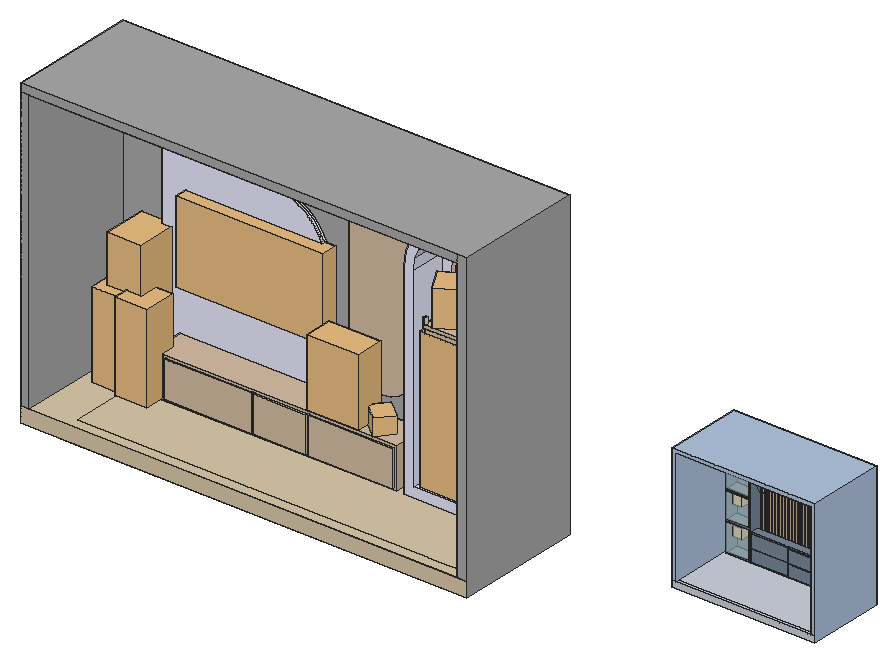
# SketchUp Ruby script. Lengths in inches.
U = 1.inch
M = Sketchup.active_model
def pt(a) = Geom::Point3d.new(a.map { |v| v * U })
def face(e, loops, mat)
  f = e.add_face(loops[0].map { |a| pt(a) })
  loops[1..].each { |l| e.add_face(l.map { |a| pt(a) }).erase! }
  f.material = f.back_material = mat if mat
  f
end
# faces: each face lists its corners as indices into pts; further lists are holes
def faces(e, pts, list, mat = nil) = list.each { |f| face(e, (f[0].is_a?(Array) ? f : [f]).map { |l| l.map { |i| pts[i] } }, mat) }
# xy, xz, yz: faces in a plane at the given z, y or x. An outline is a flat list of corners, or four numbers for a rectangle; further outlines are holes
def ring(l) = l.size == 4 ? [[l[0], l[1]], [l[2], l[1]], [l[2], l[3]], [l[0], l[3]]] : l.each_slice(2).to_a
def flat(e, list, mat, &to3) = list.each { |f| face(e, (f[0].is_a?(Array) ? f : [f]).map { |l| ring(l).map { |u, v| to3.(u, v) } }, mat) }
def xy(e, z, list, mat = nil) = flat(e, list, mat) { |x, y| [x, y, z] }
def xz(e, y, list, mat = nil) = flat(e, list, mat) { |x, z| [x, y, z] }
def yz(e, x, list, mat = nil) = flat(e, list, mat) { |y, z| [x, y, z] }
def lines(e, pts, list) = list.each { |a, b| e.add_line(pt(pts[a]), pt(pts[b])) }
# prism: a flat outline (further loops are holes) pulled along v
def prism(e, loops, v, mat = nil)
  f = face(e, loops, mat); d = Geom::Vector3d.new(v.map { |x| x * U })
  f.pushpull(f.normal.samedirection?(d) ? d.length : -d.length)
end
def box(e, o, s, mat = nil) = prism(e, [[o, [o[0] + s[0], o[1], o[2]], [o[0] + s[0], o[1] + s[1], o[2]], [o[0], o[1] + s[1], o[2]]]], [0, 0, s[2]], mat)
def at(x, y, z, deg = 0) = Geom::Transformation.translation(pt([x, y, z])) * Geom::Transformation.rotation(ORIGIN, Z_AXIS, deg.degrees)
def axes(o, x, y, z) = Geom::Transformation.new([*x, 0, *y, 0, *z, 0, *pt(o).to_a, 1])
def part(name) = M.definitions.add(name)
# library, detail: a bought-in or finely detailed component or shape, given as its bounding box
def library(name, o, s) = part(name).tap { |d| box(d.entities, o, s) }
def detail(e, o, s) = box(e.add_group.entities, o, s)
def put(e, d, t, mat = nil) = e.add_instance(d, t).tap { |i| i.material = mat if mat }
def group(e, t, mat = nil) = e.add_group.tap { |g| g.transformation = t; g.material = mat if mat }.entities
root = M.entities
M.materials.add("[0099_LightSteelBlue]").color = [176, 196, 222]
M.materials.add("[0110_LightSlateGray]").color = [119, 136, 153]
M.materials.add("[0116_Lavender]").color = [230, 230, 250]
M.materials.add("[0132_LightGray]").color = [169, 169, 169]
M.materials.add("[Field Square Tile]").color = [217, 201, 169]
M.materials.add("[Formica Laminate Light]").color = [213, 189, 164]
M.materials.add("[Marble Carrara Floor Tile]").color = [204, 208, 219]
M.materials.add("[Translucent Glass Gray]").color = [128, 128, 128]
M.materials["[Translucent Glass Gray]"].alpha = 0.5
M.materials.add("[Translucent Glass Safety]").color = [204, 235, 244]
M.materials["[Translucent Glass Safety]"].alpha = 0.5
c1 = library("Plant 260 020",[-18.86,-7.03,0.01],[33.61,20.04,67.26])
c2 = library("Potted Tree 60-30",[-14.86,-14.1,0],[27.47,27.86,74.88])
c3 = library("Books 155 025",[-5.0625,-5.83,0.01],[10.11,11.66,8.59])
c4 = library("Vase Set 001",[-13.7,-8.6,0],[27.44,16.98,21.89])
c5 = library("Seasoning Set 134 014",[-3.54,-7.03,0],[7.08,14.06,11.14])
c6 = library("Vase 20-16",[-4.28,-4.99,-0.02],[8.81,9.55,11.09])
c7 = library("Flat screen television",[0,1.41,1.14],[35.92,0.28,20.21])
c8 = library("Spot Light",[-5.1,-5.1,-11.05],[10.2,10.2,11.05])
c9 = library("Spot Light\#1",[-5.1,-5.1,-11.05],[10.2,10.2,11.05])
c10 = part("Group29\#1")
p = [[0,0,0],[0,0,-16.21],[-7.97,0,-16.21],[51.88,-0.6,0],[-51.88,-0.6,0],[51.88,0.6,0],
  [51.88,0,0],[-51.88,0.6,0],[7.97,0,-16.21],[-51.88,0,0],[0,0,-26.24]]
lines(c10.entities,p,[[0,1],[1,2],[3,4],[5,6],[7,5],[1,8],[9,0],[0,6],[8,10],[4,9],[6,3],[2,10],
  [9,7]])
c11 = part("Rectangle Light")
put(c11.entities,c10,at(0,0,0))
c12 = part("Group31\#1")
p = [[0,0,0],[0,0,-16.22],[-7.97,0,-16.22],[51.88,-0.61,0],[-51.88,-0.61,0],[51.88,0.61,0],
  [51.88,0,0],[-51.88,0.61,0],[7.97,0,-16.22],[-51.88,0,0],[0,0,-26.25]]
lines(c12.entities,p,[[0,1],[1,2],[3,4],[5,6],[7,5],[1,8],[9,0],[0,6],[8,10],[4,9],[6,3],[2,10],
  [9,7]])
c13 = part("Rectangle Light\#1")
put(c13.entities,c12,at(0,0,0))
c14 = library("Group\#6",[0,0,0],[89.875,32.5,157.0625])
xy(root,0,[[45.1875,0,502.8125,144.8125],[630.76,128.14,791.01,214.96]])
xy(root,6.6875,[[672.39,206.38,674.13,208.57],[679.86,206.38,681.61,208.57],[683.6,206.38,685.34,208.57],[687.34,206.38,689.08,208.57],[691.08,206.38,692.82,208.57],
  [694.8125,206.38,696.56,208.57],[698.55,206.38,700.3,208.57],[702.29,206.38,704.03,208.57],[706.03,206.38,707.77,208.57],[709.77,206.38,711.51,208.57],
  [713.5,206.38,715.25,208.57],[717.24,206.38,718.99,208.57],[720.98,206.38,722.73,208.57],[724.72,206.38,726.46,208.57],[728.46,206.38,730.2,208.57],
  [732.19,206.38,733.94,208.57],[735.93,206.38,737.68,208.57],[739.67,206.38,741.42,208.57],[743.41,206.38,745.15,208.57],[747.15,206.38,748.89,208.57]])
xy(root,6.6875,[[676.125,206.38,677.87,208.57]],"[Formica Laminate Light]")
xy(root,6.6875,[[634.65,128.14,787.12,132.03],[634.65,132.03,787.12,132.03,787.12,207.44,785.12,207.44,785.12,195.76,636.65,195.76,636.65,207.44,634.65,207.44],[665.65,205.5,750.99,205.5,750.99,207.44,748.89,207.44,748.89,206.38,747.15,206.38,747.15,207.44,745.15,207.44,745.15,206.38,743.41,206.38,743.41,207.44,741.42,207.44,741.42,206.38,739.67,206.38,739.67,207.44,737.68,207.44,737.68,206.38,735.93,206.38,735.93,207.44,733.94,207.44,733.94,206.38,732.19,206.38,732.19,207.44,730.2,207.44,730.2,206.38,728.46,206.38,728.46,207.44,726.46,207.44,726.46,206.38,724.72,206.38,724.72,207.44,722.73,207.44,722.73,206.38,720.98,206.38,720.98,207.44,718.99,207.44,718.99,206.38,717.24,206.38,717.24,207.44,715.25,207.44,715.25,206.38,713.5,206.38,713.5,207.44,711.51,207.44,711.51,206.38,709.77,206.38,709.77,207.44,707.77,207.44,707.77,206.38,706.03,206.38,706.03,207.44,704.03,207.44,704.03,206.38,702.29,206.38,702.29,207.44,700.3,207.44,700.3,206.38,698.55,206.38,698.55,207.44,696.56,207.44,696.56,206.38,694.8125,206.38,694.8125,207.44,692.82,207.44,692.82,206.38,691.08,206.38,691.08,207.44,689.08,207.44,689.08,206.38,687.34,206.38,687.34,207.44,685.34,207.44,685.34,206.38,683.6,206.38,683.6,207.44,681.61,207.44,681.61,206.38,679.86,206.38,679.86,207.44,677.87,207.44,677.87,206.38,676.125,206.38,676.125,207.44,674.13,207.44,674.13,206.38,672.39,206.38,672.39,207.44,670.39,207.44,670.39,206.38,668.65,206.38,668.65,207.44,665.65,207.44]],"[Marble Carrara Floor Tile]")
xy(root,8.46,[[665.65,194.69,707.33,195.76],[707.83,194.69,750.9,195.76],[638.42,195.76,663.88,209.51]],"[0110_LightSlateGray]")
xy(root,8.46,[[638.42,194.26,663.88,195.76]],"[Translucent Glass Safety]")
xy(root,9.53,[[753.9,195.76,782.28,208.32]],"[0110_LightSlateGray]")
xy(root,9.53,[[753.9,193.44,782.28,195.76]],"[Translucent Glass Safety]")
xy(root,16.875,[[78.33,87.35,78.33,126.85,57.15,126.85,57.15,129.85,244.65,129.85,244.65,126.85,353.21,126.85,353.21,87.35],[361.77,87.35,480.71,90.35],[361.77,90.35,480.71,132.85],[57.15,129.85,244.65,132.85]])
xy(root,21.55,[[665.65,194.69,707.33,195.76],[707.83,194.69,750.9,195.76]],"[0110_LightSlateGray]")
xy(root,22.05,[[665.65,194.69,707.33,195.76],[707.83,194.69,750.9,195.76]],"[0110_LightSlateGray]")
xy(root,27.89,[[[372.78,87.35,469.7,126.35],[376.68,90.54,466.56,123.04]]],"[0116_Lavender]")
xy(root,36.6875,[[665.65,194.69,707.33,195.76],[707.83,194.69,750.9,195.76]],"[0110_LightSlateGray]")
xy(root,38,[[665.65,195.76,750.99,205.5]],"[0110_LightSlateGray]")
xy(root,39.67,[[638.42,195.76,663.88,209.51]],"[0110_LightSlateGray]")
xy(root,39.67,[[638.42,194.26,663.88,195.76]],"[Translucent Glass Safety]")
xy(root,40.2,[[753.9,195.76,782.28,208.32]],"[0110_LightSlateGray]")
xy(root,40.2,[[753.9,193.44,782.28,195.76]],"[Translucent Glass Safety]")
xy(root,41.68,[[638.42,194.26,663.88,195.76]],"[Translucent Glass Gray]")
xy(root,42.2,[[753.9,195.76,782.28,208.32]],"[0110_LightSlateGray]")
xy(root,42.2,[[753.9,193.44,782.28,195.76]],"[Translucent Glass Gray]")
xy(root,70.875,[[638.42,195.76,663.88,209.51],[753.9,195.76,782.28,208.32]],"[0110_LightSlateGray]")
xy(root,70.875,[[753.9,193.44,782.28,195.76],[638.42,194.26,663.88,195.76]],"[Translucent Glass Safety]")
xy(root,72.875,[[638.42,194.26,663.88,195.76]])
xy(root,72.875,[[638.42,195.76,663.88,209.51],[753.9,195.76,782.28,208.32]],"[0110_LightSlateGray]")
xy(root,72.875,[[753.9,193.44,782.28,195.76]],"[Translucent Glass Safety]")
xy(root,101.55,[[753.9,195.76,782.28,208.32]],"[0110_LightSlateGray]")
xy(root,101.55,[[753.9,193.44,782.28,195.76]],"[Translucent Glass Safety]")
xy(root,102.08,[[638.42,195.76,663.88,209.51]],"[0110_LightSlateGray]")
xy(root,102.08,[[638.42,194.26,663.88,195.76]],"[Translucent Glass Safety]")
xy(root,103.55,[[753.9,195.76,782.28,208.32]],"[0110_LightSlateGray]")
xy(root,103.55,[[753.9,193.44,782.28,195.76]],"[Translucent Glass Safety]")
xy(root,104.08,[[638.42,195.76,663.88,209.51]],"[0110_LightSlateGray]")
xy(root,104.08,[[638.42,194.26,663.88,195.76]],"[Translucent Glass Gray]")
xy(root,132.22,[[753.9,195.76,782.28,208.32]],"[0110_LightSlateGray]")
xy(root,132.22,[[753.9,193.44,782.28,195.76]],"[Translucent Glass Safety]")
xy(root,133.29,[[638.42,194.26,663.88,195.76]])
xy(root,133.29,[[638.42,195.76,663.88,209.51]],"[0110_LightSlateGray]")
xy(root,135.0625,[[636.65,195.76,665.65,207.44],[750.99,195.76,785.12,207.44],[668.65,206.38,670.39,207.44],[672.39,206.38,674.13,207.44],[676.125,206.38,677.87,207.44],
  [679.86,206.38,681.61,207.44],[683.6,206.38,685.34,207.44],[687.34,206.38,689.08,207.44],[691.08,206.38,692.82,207.44],[694.8125,206.38,696.56,207.44],
  [698.55,206.38,700.3,207.44],[702.29,206.38,704.03,207.44],[706.03,206.38,707.77,207.44],[709.77,206.38,711.51,207.44],[713.5,206.38,715.25,207.44],
  [717.24,206.38,718.99,207.44],[720.98,206.38,722.73,207.44],[724.72,206.38,726.46,207.44],[728.46,206.38,730.2,207.44],[732.19,206.38,733.94,207.44],
  [735.93,206.38,737.68,207.44],[739.67,206.38,741.42,207.44],[743.41,206.38,745.15,207.44],[747.15,206.38,748.89,207.44]])
xy(root,136.0625,[[[634.65,128.14,787.12,207.44],[659,152.5,762.77,184.22]],[[660.14,153.63,761.63,183.08],[664.93,158.43,756.83,178.28]],[665.63,159.13,756.13,177.58]],"[0099_LightSteelBlue]")
xy(root,136.5625,[[[664.93,158.43,756.83,178.28],[665.63,159.13,756.13,177.58]]],"[0099_LightSteelBlue]")
xy(root,136.9375,[[[659,152.5,762.77,184.22],[660.14,153.63,761.63,183.08]]],"[0099_LightSteelBlue]")
xy(root,140.25,[[630.76,128.14,791.01,214.96]],"[0099_LightSteelBlue]")
xy(root,190.07,[[380.12,90.54,462.49,123.04]])
xy(root,193.2,[[383.06,90.54,459.87,123.04],[380.12,94.54,383.06,123.04],[459.87,94.54,462.49,123.04]],"[Formica Laminate Light]")
xy(root,200.39,[[380.12,90.54,383.06,94.54],[459.87,90.54,462.49,94.54]],"[Formica Laminate Light]")
xy(root,247.25,[[57.15,129.85,176.83,132.85]])
xy(root,314.3125,[[272.9,124.42,347.58,132.85]])
xz(root,87.35,[[[361.77,16.875,480.71,16.875,480.71,247.25,478.68,262.64,472.74,276.98,463.29,289.3,450.97,298.75,436.63,304.69,421.24,306.72,405.85,304.69,391.51,298.75,379.1875,289.3,369.74,276.98,363.8,262.64,361.77,247.25],[372.78,27.89,372.78,247.25,374.43,259.79,379.27,271.48,386.98,281.51,397.01,289.22,408.7,294.06,421.24,295.71,433.78,294.06,445.47,289.22,455.5,281.51,463.21,271.48,468.05,259.79,469.7,247.25,469.7,27.89]]],"[0116_Lavender]")
xz(root,90.54,[[380.12,190.07,462.49,190.07,462.49,200.39,459.87,200.39,459.87,193.2,383.06,193.2,383.06,200.39,380.12,200.39]],"[Formica Laminate Light]")
xz(root,94.54,[[380.12,193.2,383.06,200.39],[459.87,193.2,462.49,200.39]])
xz(root,121.42,[[310.24,84.22,319.91,85.49,328.91,89.22,336.65,95.16,342.58,102.89,346.3125,111.9,347.58,121.57,347.58,314.3125,272.9,314.3125,272.9,121.57,274.17,111.9,277.9,102.89,283.83,95.16,291.57,89.22,300.57,85.49]],"[Formica Laminate Light]")
xz(root,123.04,[[376.68,27.89,376.68,178.07,376.73,178.93,376.89,179.77,377.16,180.59,377.52,181.37,377.98,182.1,378.52,182.76,379.14,183.35,379.83,183.86,380.58,184.28,381.375,184.61,382.2,184.83,383.06,184.95,383.06,190.07,380.12,190.07,380.12,193.2,462.49,193.2,462.49,190.07,459.87,190.07,459.87,184.95,460.74,184.89,461.6,184.72,462.43,184.44,463.21,184.05,463.9375,183.57,464.6,182.99,465.17,182.33,465.66,181.61,466.05,180.82,466.33,179.99,466.5,179.13,466.56,178.26,466.56,27.89]],"[0116_Lavender]")
xz(root,126.35,[[[372.78,27.89,469.7,27.89,469.7,247.25,468.05,259.79,463.21,271.48,455.5,281.51,445.47,289.22,433.78,294.06,421.24,295.71,408.7,294.06,397.01,289.22,386.98,281.51,379.27,271.48,374.43,259.79,372.78,247.25],[420.74,196.23,410.97,197.97,401.99,202.17,394.4,208.5625,388.72,216.7,385.35,226.03,384.5,235.91,386.24,245.68,390.44,254.66,396.83,262.25,404.97,267.93,414.29,271.3,424.18,272.15,433.94,270.41,442.93,266.21,450.52,259.82,456.19,251.68,459.57,242.35,460.42,232.47,458.68,222.7,454.47,213.72,448.09,206.13,439.95,200.46,430.62,197.08]],[[420.875,199.21,429.98,199.99,438.58,203.1,446.08,208.33,451.96,215.33,455.84,223.61,457.44,232.61,456.66,241.71,453.55,250.31,448.32,257.81,441.32,263.7,433.04,267.57,424.04,269.17,414.93,268.39,406.34,265.28,398.84,260.05,392.95,253.05,389.08,244.78,387.47,235.77,388.26,226.67,391.37,218.07,396.6,210.57,403.59,204.69,411.875,200.81],[423.06,204.82,415.4375,205.67,408.3,208.46,402.12,213,397.33,218.98,394.25,226.01,393.09,233.59,393.93,241.21,396.72,248.35,401.27,254.53,407.25,259.32,414.28,262.4,421.86,263.56,429.48,262.71,436.62,259.93,442.8,255.38,447.59,249.4,450.67,242.37,451.83,234.79,450.98,227.17,448.19,220.03,443.65,213.85,437.66,209.06,430.64,205.98]]],"[0116_Lavender]")
xz(root,126.35,[[[420.74,196.23,430.62,197.08,439.95,200.46,448.09,206.13,454.47,213.72,458.68,222.7,460.42,232.47,459.57,242.35,456.19,251.68,450.52,259.82,442.93,266.21,433.94,270.41,424.18,272.15,414.29,271.3,404.97,267.93,396.83,262.25,390.44,254.66,386.24,245.68,384.5,235.91,385.35,226.03,388.72,216.7,394.4,208.5625,401.99,202.17,410.97,197.97],[420.875,199.21,411.875,200.81,403.59,204.69,396.6,210.57,391.37,218.07,388.26,226.67,387.47,235.77,389.08,244.78,392.95,253.05,398.84,260.05,406.34,265.28,414.93,268.39,424.04,269.17,433.04,267.57,441.32,263.7,448.32,257.81,453.55,250.31,456.66,241.71,457.44,232.61,455.84,223.61,451.96,215.33,446.08,208.33,438.58,203.1,429.98,199.99]],[423.06,204.82,430.64,205.98,437.66,209.06,443.65,213.85,448.19,220.03,450.98,227.17,451.83,234.79,450.67,242.37,447.59,249.4,442.8,255.38,436.62,259.93,429.48,262.71,421.86,263.56,414.28,262.4,407.25,259.32,401.27,254.53,396.72,248.35,393.93,241.21,393.09,233.59,394.25,226.01,397.33,218.98,402.12,213,408.3,208.46,415.4375,205.67]],"[Formica Laminate Light]")
xz(root,126.85,[[244.65,16.875,353.21,62.4375]])
xz(root,126.85,[[57.15,16.875,78.33,16.875,78.33,62.4375,244.65,62.4375,244.65,179.43,244.07,188.28,242.34,196.98,239.48,205.38,235.56,213.34,230.63,220.72,224.78,227.39,218.11,233.24,210.74,238.16,202.78,242.09,194.38,244.9375,185.68,246.67,176.83,247.25,57.15,247.25]],"[0116_Lavender]")
xz(root,128.14,[[630.76,6.6875,634.65,6.6875,634.65,136.0625,787.12,136.0625,787.12,6.6875,791.01,6.6875,791.01,140.25,630.76,140.25]],"[0099_LightSteelBlue]")
xz(root,128.14,[[630.76,0,791.01,6.6875]],"[Marble Carrara Floor Tile]")
xz(root,132.85,[[57.15,16.875,57.15,247.25,176.83,247.25,185.68,246.67,194.38,244.9375,202.78,242.09,210.74,238.16,218.11,233.24,224.78,227.39,230.63,220.72,235.56,213.34,239.48,205.38,242.34,196.98,244.07,188.28,244.65,179.43,244.65,16.875],[361.77,16.875,361.77,247.25,363.8,262.64,369.74,276.98,379.1875,289.3,391.51,298.75,405.85,304.69,421.24,306.72,436.63,304.69,450.97,298.75,463.29,289.3,472.74,276.98,478.68,262.64,480.71,247.25,480.71,16.875],[310.24,84.22,300.57,85.49,291.57,89.22,283.83,95.16,277.9,102.89,274.17,111.9,272.9,121.57,272.9,314.3125,347.58,314.3125,347.58,121.57,346.3125,111.9,342.58,102.89,336.65,95.16,328.91,89.22,319.91,85.49]])
xz(root,152.5,[[659,136.0625,762.77,136.9375]],"[0099_LightSteelBlue]")
xz(root,153.63,[[660.14,136.0625,761.63,136.9375]],"[0099_LightSteelBlue]")
xz(root,158.43,[[664.93,136.0625,756.83,136.5625]],"[0099_LightSteelBlue]")
xz(root,159.13,[[665.63,136.0625,756.13,136.5625]],"[0099_LightSteelBlue]")
xz(root,177.58,[[665.63,136.0625,756.13,136.5625]],"[0099_LightSteelBlue]")
xz(root,178.28,[[664.93,136.0625,756.83,136.5625]],"[0099_LightSteelBlue]")
xz(root,183.08,[[660.14,136.0625,761.63,136.9375]],"[0099_LightSteelBlue]")
xz(root,184.22,[[659,136.0625,762.77,136.9375]],"[0099_LightSteelBlue]")
xz(root,193.44,[[753.9,9.53,782.28,40.2],[753.9,42.2,782.28,70.875],[753.9,72.875,782.28,101.55],[753.9,103.55,782.28,132.22]],"[Translucent Glass Safety]")
xz(root,194.26,[[638.42,8.46,663.88,39.67],[638.42,41.68,663.88,70.875],[638.42,72.875,663.88,102.08],[638.42,104.08,663.88,133.29]],"[Translucent Glass Safety]")
xz(root,194.69,[[665.65,8.46,707.33,21.55],[707.83,8.46,750.9,21.55],[665.65,22.05,707.33,36.6875],[707.83,22.05,750.9,36.6875]],"[0110_LightSlateGray]")
xz(root,195.76,[[[636.65,6.6875,785.12,6.6875,785.12,135.0625,750.99,135.0625,750.99,38,665.65,38,665.65,135.0625,636.65,135.0625],[753.9,9.53,782.28,132.22],[638.42,8.46,663.88,133.29],[707.83,22.05,750.9,36.6875],[665.65,22.05,707.33,36.6875],[707.83,8.46,750.9,21.55],[665.65,8.46,707.33,21.55]],[638.42,39.67,663.88,41.68],[753.9,40.2,782.28,42.2],[638.42,70.875,663.88,72.875],[753.9,70.875,782.28,72.875],
  [753.9,101.55,782.28,103.55],[638.42,102.08,663.88,104.08]],"[0110_LightSlateGray]")
xz(root,205.5,[[665.65,6.6875,750.99,38]],"[0110_LightSlateGray]")
xz(root,206.38,[[668.65,6.6875,670.39,135.0625],[672.39,6.6875,674.13,135.0625],[676.125,6.6875,677.87,135.0625],[679.86,6.6875,681.61,135.0625],[683.6,6.6875,685.34,135.0625],
  [687.34,6.6875,689.08,135.0625],[691.08,6.6875,692.82,135.0625],[694.8125,6.6875,696.56,135.0625],[698.55,6.6875,700.3,135.0625],[702.29,6.6875,704.03,135.0625],
  [706.03,6.6875,707.77,135.0625],[709.77,6.6875,711.51,135.0625],[713.5,6.6875,715.25,135.0625],[717.24,6.6875,718.99,135.0625],[720.98,6.6875,722.73,135.0625],
  [724.72,6.6875,726.46,135.0625],[728.46,6.6875,730.2,135.0625],[732.19,6.6875,733.94,135.0625],[735.93,6.6875,737.68,135.0625],[739.67,6.6875,741.42,135.0625],
  [743.41,6.6875,745.15,135.0625],[747.15,6.6875,748.89,135.0625]],"[Formica Laminate Light]")
xz(root,207.44,[[634.65,6.6875,636.65,6.6875,636.65,135.0625,665.65,135.0625,665.65,6.6875,668.65,6.6875,668.65,135.0625,670.39,135.0625,670.39,6.6875,672.39,6.6875,672.39,135.0625,674.13,135.0625,674.13,6.6875,676.125,6.6875,676.125,135.0625,677.87,135.0625,677.87,6.6875,679.86,6.6875,679.86,135.0625,681.61,135.0625,681.61,6.6875,683.6,6.6875,683.6,135.0625,685.34,135.0625,685.34,6.6875,687.34,6.6875,687.34,135.0625,689.08,135.0625,689.08,6.6875,691.08,6.6875,691.08,135.0625,692.82,135.0625,692.82,6.6875,694.8125,6.6875,694.8125,135.0625,696.56,135.0625,696.56,6.6875,698.55,6.6875,698.55,135.0625,700.3,135.0625,700.3,6.6875,702.29,6.6875,702.29,135.0625,704.03,135.0625,704.03,6.6875,706.03,6.6875,706.03,135.0625,707.77,135.0625,707.77,6.6875,709.77,6.6875,709.77,135.0625,711.51,135.0625,711.51,6.6875,713.5,6.6875,713.5,135.0625,715.25,135.0625,715.25,6.6875,717.24,6.6875,717.24,135.0625,718.99,135.0625,718.99,6.6875,720.98,6.6875,720.98,135.0625,722.73,135.0625,722.73,6.6875,724.72,6.6875,724.72,135.0625,726.46,135.0625,726.46,6.6875,728.46,6.6875,728.46,135.0625,730.2,135.0625,730.2,6.6875,732.19,6.6875,732.19,135.0625,733.94,135.0625,733.94,6.6875,735.93,6.6875,735.93,135.0625,737.68,135.0625,737.68,6.6875,739.67,6.6875,739.67,135.0625,741.42,135.0625,741.42,6.6875,743.41,6.6875,743.41,135.0625,745.15,135.0625,745.15,6.6875,747.15,6.6875,747.15,135.0625,748.89,135.0625,748.89,6.6875,750.99,6.6875,750.99,135.0625,785.12,135.0625,785.12,6.6875,787.12,6.6875,787.12,136.0625,634.65,136.0625]],"[0099_LightSteelBlue]")
xz(root,208.32,[[753.9,9.53,782.28,40.2],[753.9,42.2,782.28,70.875],[753.9,72.875,782.28,101.55],[753.9,103.55,782.28,132.22]],"[0110_LightSlateGray]")
xz(root,209.51,[[638.42,8.46,663.88,39.67],[638.42,41.67,663.88,70.875],[638.42,72.875,663.88,102.08],[638.42,104.08,663.88,133.29]],"[0110_LightSlateGray]")
xz(root,214.96,[[630.76,0,791.01,140.25]])
yz(root,57.15,[[129.85,16.875,132.85,247.25]])
yz(root,244.65,[[129.85,16.875,132.85,179.43]])
yz(root,272.9,[[124.42,121.57,132.85,314.3125]],"[Formica Laminate Light]")
yz(root,347.58,[[124.42,121.57,132.85,314.3125]])
yz(root,361.77,[[90.35,16.875,132.85,247.25]],"[0116_Lavender]")
yz(root,372.78,[[87.35,27.89,126.35,247.25]],"[0116_Lavender]")
yz(root,380.12,[[90.54,190.07,90.54,200.39,94.54,200.39,94.54,193.2,123.04,193.2,123.04,190.07]],"[Formica Laminate Light]")
yz(root,383.06,[[90.54,193.2,94.54,200.39]])
yz(root,459.87,[[90.54,193.2,94.54,200.39]],"[Formica Laminate Light]")
yz(root,462.49,[[90.54,190.07,123.04,190.07,123.04,193.2,94.54,193.2,94.54,200.39,90.54,200.39]])
yz(root,469.7,[[87.35,27.89,126.35,247.25]],"[0116_Lavender]")
yz(root,480.71,[[90.35,16.875,132.85,247.25]])
yz(root,630.76,[[128.14,0,214.96,140.25]],"[0099_LightSteelBlue]")
yz(root,634.65,[[128.14,6.6875,207.44,136.0625]],"[0099_LightSteelBlue]")
yz(root,636.65,[[195.76,6.6875,207.44,135.0625]])
yz(root,638.42,[[195.76,8.46,209.51,39.67],[209.51,41.67,209.51,70.875,195.76,70.875,195.76,41.68],[195.76,72.875,209.51,102.08],[195.76,104.08,209.51,133.29]],"[0110_LightSlateGray]")
yz(root,638.42,[[194.26,8.46,195.76,39.67],[194.26,41.68,195.76,70.875],[194.26,72.875,195.76,102.08],[194.26,104.08,195.76,133.29]],"[Translucent Glass Safety]")
yz(root,659,[[152.5,136.0625,184.22,136.9375]],"[0099_LightSteelBlue]")
yz(root,660.14,[[153.63,136.0625,183.08,136.9375]],"[0099_LightSteelBlue]")
yz(root,663.88,[[195.76,39.67,209.51,39.67,209.51,41.67,195.76,41.68],[195.76,70.875,209.51,72.875],[195.76,102.08,209.51,104.08]])
yz(root,663.88,[[195.76,8.46,209.51,39.67],[209.51,41.67,195.76,41.68,195.76,70.875,209.51,70.875],[195.76,104.08,209.51,133.29]],"[0110_LightSlateGray]")
yz(root,663.88,[[195.76,72.875,209.51,102.08]],"[Translucent Glass Gray]")
yz(root,663.88,[[194.26,8.46,195.76,39.67],[194.26,41.68,195.76,70.875],[194.26,72.875,195.76,102.08],[194.26,104.08,195.76,133.29]],"[Translucent Glass Safety]")
yz(root,664.93,[[158.43,136.0625,178.28,136.5625]],"[0099_LightSteelBlue]")
yz(root,665.63,[[159.13,136.0625,177.58,136.5625]],"[0099_LightSteelBlue]")
yz(root,665.65,[[206.61,6.6875,207.44,6.6875,207.44,135.0625,195.76,135.0625,195.76,38,205.5,38,205.5,29.0625,206.61,29.0625],[205.5,6.6875,206.61,29.0625],[194.69,8.46,195.76,21.55],[194.69,22.05,195.76,36.6875]],"[0110_LightSlateGray]")
yz(root,668.65,[[206.38,6.6875,207.44,135.0625]])
yz(root,670.39,[[206.38,6.6875,207.44,135.0625]],"[Formica Laminate Light]")
yz(root,672.39,[[206.38,6.6875,207.44,135.0625]],"[Formica Laminate Light]")
yz(root,674.13,[[206.38,6.6875,207.44,135.0625]],"[Formica Laminate Light]")
yz(root,676.125,[[206.38,6.6875,207.44,135.0625]],"[Formica Laminate Light]")
yz(root,677.87,[[206.38,6.6875,207.44,135.0625]],"[Formica Laminate Light]")
yz(root,679.86,[[206.38,6.6875,207.44,135.0625]],"[Formica Laminate Light]")
yz(root,681.61,[[206.38,6.6875,207.44,135.0625]],"[Formica Laminate Light]")
yz(root,683.6,[[206.38,6.6875,207.44,135.0625]],"[Formica Laminate Light]")
yz(root,685.34,[[206.38,6.6875,207.44,135.0625]],"[Formica Laminate Light]")
yz(root,687.34,[[206.38,6.6875,207.44,135.0625]],"[Formica Laminate Light]")
yz(root,689.08,[[206.38,6.6875,207.44,135.0625]],"[Formica Laminate Light]")
yz(root,691.08,[[206.38,6.6875,207.44,135.0625]],"[Formica Laminate Light]")
yz(root,692.82,[[206.38,6.6875,207.44,135.0625]],"[Formica Laminate Light]")
yz(root,694.8125,[[206.38,6.6875,207.44,135.0625]],"[Formica Laminate Light]")
yz(root,696.56,[[206.38,6.6875,207.44,135.0625]],"[Formica Laminate Light]")
yz(root,698.55,[[206.38,6.6875,207.44,135.0625]],"[Formica Laminate Light]")
yz(root,700.3,[[206.38,6.6875,207.44,135.0625]],"[Formica Laminate Light]")
yz(root,702.29,[[206.38,6.6875,207.44,135.0625]],"[Formica Laminate Light]")
yz(root,704.03,[[206.38,6.6875,207.44,135.0625]],"[Formica Laminate Light]")
yz(root,706.03,[[206.38,6.6875,207.44,135.0625]],"[Formica Laminate Light]")
yz(root,707.33,[[194.69,8.46,195.76,21.55],[194.69,22.05,195.76,36.6875]],"[0110_LightSlateGray]")
yz(root,707.77,[[206.38,6.6875,207.44,135.0625]],"[Formica Laminate Light]")
yz(root,707.83,[[194.69,8.46,195.76,21.55],[194.69,22.05,195.76,36.6875]],"[0110_LightSlateGray]")
yz(root,709.77,[[206.38,6.6875,207.44,135.0625]],"[Formica Laminate Light]")
yz(root,711.51,[[206.38,6.6875,207.44,135.0625]],"[Formica Laminate Light]")
yz(root,713.5,[[206.38,6.6875,207.44,135.0625]],"[Formica Laminate Light]")
yz(root,715.25,[[206.38,6.6875,207.44,135.0625]],"[Formica Laminate Light]")
yz(root,717.24,[[206.38,6.6875,207.44,135.0625]],"[Formica Laminate Light]")
yz(root,718.99,[[206.38,6.6875,207.44,135.0625]],"[Formica Laminate Light]")
yz(root,720.98,[[206.38,6.6875,207.44,135.0625]],"[Formica Laminate Light]")
yz(root,722.73,[[206.38,6.6875,207.44,135.0625]],"[Formica Laminate Light]")
yz(root,724.72,[[206.38,6.6875,207.44,135.0625]],"[Formica Laminate Light]")
yz(root,726.46,[[206.38,6.6875,207.44,135.0625]],"[Formica Laminate Light]")
yz(root,728.46,[[206.38,6.6875,207.44,135.0625]],"[Formica Laminate Light]")
yz(root,730.2,[[206.38,6.6875,207.44,135.0625]],"[Formica Laminate Light]")
yz(root,732.19,[[206.38,6.6875,207.44,135.0625]],"[Formica Laminate Light]")
yz(root,733.94,[[206.38,6.6875,207.44,135.0625]],"[Formica Laminate Light]")
yz(root,735.93,[[206.38,6.6875,207.44,135.0625]],"[Formica Laminate Light]")
yz(root,737.68,[[206.38,6.6875,207.44,135.0625]],"[Formica Laminate Light]")
yz(root,739.67,[[206.38,6.6875,207.44,135.0625]],"[Formica Laminate Light]")
yz(root,741.42,[[206.38,6.6875,207.44,135.0625]],"[Formica Laminate Light]")
yz(root,743.41,[[206.38,6.6875,207.44,135.0625]],"[Formica Laminate Light]")
yz(root,745.15,[[206.38,6.6875,207.44,135.0625]],"[Formica Laminate Light]")
yz(root,747.15,[[206.38,6.6875,207.44,135.0625]],"[Formica Laminate Light]")
yz(root,748.89,[[206.38,6.6875,207.44,135.0625]],"[Formica Laminate Light]")
yz(root,750.9,[[194.69,8.46,195.76,21.55],[194.69,22.05,195.76,36.6875]],"[0110_LightSlateGray]")
yz(root,750.99,[[205.5,6.6875,205.5,38,195.76,38,195.76,135.0625,207.44,135.0625,207.44,6.6875]],"[0110_LightSlateGray]")
yz(root,753.9,[[195.76,9.53,208.32,40.2],[195.76,42.2,208.32,70.875],[195.76,72.875,208.32,101.55],[195.76,103.55,208.32,132.22]],"[0110_LightSlateGray]")
yz(root,753.9,[[193.44,9.53,195.76,40.2],[193.44,42.2,195.76,70.875],[193.44,72.875,195.76,101.55],[193.44,103.55,195.76,132.22]],"[Translucent Glass Safety]")
yz(root,756.13,[[159.13,136.0625,177.58,136.5625]],"[0099_LightSteelBlue]")
yz(root,756.83,[[158.43,136.0625,178.28,136.5625]],"[0099_LightSteelBlue]")
yz(root,761.63,[[153.63,136.0625,183.08,136.9375]],"[0099_LightSteelBlue]")
yz(root,762.77,[[152.5,136.0625,184.22,136.9375]],"[0099_LightSteelBlue]")
yz(root,782.28,[[195.76,40.2,208.32,42.2],[195.76,70.875,208.32,72.875],[195.76,101.55,208.32,103.55]])
yz(root,782.28,[[195.76,9.53,208.32,40.2],[195.76,42.2,208.32,70.875],[195.76,72.875,208.32,101.55],[195.76,103.55,208.32,132.22]],"[0110_LightSlateGray]")
yz(root,782.28,[[193.44,9.53,195.76,40.2],[193.44,42.2,195.76,70.875],[193.44,72.875,195.76,101.55],[193.44,103.55,195.76,132.22]],"[Translucent Glass Safety]")
yz(root,785.12,[[195.76,6.6875,207.44,135.0625]])
yz(root,787.12,[[128.14,6.6875,207.44,136.0625]],"[0099_LightSteelBlue]")
yz(root,791.01,[[128.14,0,214.96,140.25]],"[0099_LightSteelBlue]")
p = [[638.42,209.51,41.67],[638.42,195.76,41.68],[663.88,195.76,41.68],[663.88,209.51,41.67],[310.24,132.85,84.22],[310.24,124.42,84.22],
  [300.57,124.42,85.49],[300.57,132.85,85.49],[319.91,132.85,85.49],[319.91,124.42,85.49],[291.57,124.42,89.22],[291.57,132.85,89.22],
  [328.91,132.85,89.22],[328.91,124.42,89.22],[283.83,124.42,95.16],[283.83,132.85,95.16],[336.65,132.85,95.16],[336.65,124.42,95.16],
  [277.9,124.42,102.89],[277.9,132.85,102.89],[342.58,132.85,102.89],[342.58,124.42,102.89],[274.17,124.42,111.9],[274.17,132.85,111.9],
  [346.3125,132.85,111.9],[346.3125,124.42,111.9],[272.9,124.42,121.57],[272.9,132.85,121.57],[347.58,132.85,121.57],[347.58,124.42,121.57],
  [244.07,132.85,188.28],[244.07,129.85,188.28],[244.65,129.85,179.43],[244.65,132.85,179.43],[242.34,132.85,196.98],[242.34,129.85,196.98],
  [239.48,132.85,205.38],[239.48,129.85,205.38],[235.56,132.85,213.34],[235.56,129.85,213.34],[230.63,132.85,220.72],[230.63,129.85,220.72],
  [224.78,132.85,227.39],[224.78,129.85,227.39],[218.11,132.85,233.24],[218.11,129.85,233.24],[210.74,132.85,238.16],[210.74,129.85,238.16],
  [202.78,132.85,242.09],[202.78,129.85,242.09],[194.38,132.85,244.9375],[194.38,129.85,244.9375],[185.68,132.85,246.67],[185.68,129.85,246.67],
  [176.83,132.85,247.25],[176.83,129.85,247.25],[374.43,87.35,259.79],[372.78,87.35,247.25],[372.78,126.35,247.25],[374.43,126.35,259.79],
  [361.77,132.85,247.25],[361.77,90.35,247.25],[363.8,90.35,262.64],[363.8,132.85,262.64],[478.68,132.85,262.64],[478.68,90.35,262.64],
  [480.71,90.35,247.25],[480.71,132.85,247.25],[469.7,87.35,247.25],[468.05,87.35,259.79],[468.05,126.35,259.79],[469.7,126.35,247.25],
  [379.27,87.35,271.48],[379.27,126.35,271.48],[463.21,87.35,271.48],[463.21,126.35,271.48],[369.74,90.35,276.98],[369.74,132.85,276.98],
  [472.74,132.85,276.98],[472.74,90.35,276.98],[386.98,87.35,281.51],[386.98,126.35,281.51],[455.5,87.35,281.51],[455.5,126.35,281.51],
  [379.1875,90.35,289.3],[379.1875,132.85,289.3],[463.29,132.85,289.3],[463.29,90.35,289.3],[397.01,87.35,289.22],[397.01,126.35,289.22],
  [445.47,87.35,289.22],[445.47,126.35,289.22],[408.7,87.35,294.06],[408.7,126.35,294.06],[433.78,87.35,294.06],[433.78,126.35,294.06],
  [391.51,90.35,298.75],[391.51,132.85,298.75],[450.97,132.85,298.75],[450.97,90.35,298.75],[421.24,87.35,295.71],[421.24,126.35,295.71],
  [405.85,90.35,304.69],[405.85,132.85,304.69],[436.63,132.85,304.69],[436.63,90.35,304.69],[421.24,90.35,306.72],[421.24,132.85,306.72]]
faces(root,p,[[0,1,2,3]],"[0110_LightSlateGray]")
faces(root,p,[[4,5,6,7],[8,9,5,4],[7,6,10,11],[12,13,9,8],[11,10,14,15],[16,17,13,12],[15,14,18,19],[20,21,17,16],
  [19,18,22,23],[24,25,21,20],[23,22,26,27],[28,29,25,24]],"[Formica Laminate Light]")
faces(root,p,[[30,31,32,33],[34,35,31,30],[36,37,35,34],[38,39,37,36],[40,41,39,38],[42,43,41,40],[44,45,43,42],[46,47,45,44],
  [48,49,47,46],[50,51,49,48],[52,53,51,50],[54,55,53,52],[56,57,58,59],[60,61,62,63],[64,65,66,67],[68,69,70,71],
  [72,56,59,73],[69,74,75,70],[63,62,76,77],[78,79,65,64],[80,72,73,81],[74,82,83,75],[77,76,84,85],[86,87,79,78],
  [88,80,81,89],[82,90,91,83],[92,88,89,93],[90,94,95,91],[85,84,96,97],[98,99,87,86],[100,92,93,101],[94,100,101,95],
  [97,96,102,103],[104,105,99,98],[103,102,106,107],[107,106,105,104]],"[0116_Lavender]")
put(root,c1,axes([51.93,100.98,16.86],[1.15,0,0],[0,2.45008,0],[0,0,2.2176]))
put(root,c2,axes([41.11,90.77,16.875],[1.29,0,0],[0,1.29,0],[0,0,1.29]))
put(root,c2,axes([71.97,85.92,16.78],[1.32,0,0],[0,1.32,0],[0,0,1.32]))
put(root,c3,axes([323.45,103.93,62.41],[1.37487,1.69178,0],[-1.69178,1.37487,0],[0,0,2.18]))
put(root,c4,axes([280.32,104.84,62.44],[2.139,0,0],[0,1.86,0],[0,0,3.4596]))
put(root,c5,axes([392.11,109.48,193.05],[2.69266,1.55461,0],[-1.13475,1.96544,0],[0,0,3.6085]))
put(root,c6,axes([441.9,107.11,193.24],[2.93872,0,0],[0,2.2263,0],[0,0,3.33945]))
put(root,c7,axes([84.56,21.71,111.98],[4.62917,0,0],[0,64.40536,0],[0,0,4.5384]))
put(root,c8,at(650.91,200.11,131.72))
put(root,c8,at(650.91,200.11,102.08))
put(root,c8,at(650.91,200.11,70.875))
put(root,c8,at(650.91,200.11,38.25))
put(root,c9,at(767.8,199.45,130.59))
put(root,c9,at(767.8,199.45,98.65))
put(root,c9,at(767.8,197.81,69.5))
put(root,c9,at(768.69,201.1875,38.2))
put(root,c11,axes([710.88,153.06,136.0625],[1,0,0],[0,0.94478,0],[0,0,1.00038]))
put(root,c13,axes([710.88,183.65,136.0625],[1,0,0],[0,0.92658,0],[0,0,1.00038]))
g1 = group(root,at(45.1875,0,0),"[0132_LightGray]")
xy(g1,16.875,[[-36.1875,0,445.67,0,445.67,11.96,8.96,11.96,8.96,132.85,-36.1875,132.85],[8.96,11.96,445.67,132.85]],"[Field Square Tile]")
xy(g1,333.625,[[-35.5,0,11.96,132.85]])
xy(g1,333.625,[[11.96,0,445.67,132.85]],"[0132_LightGray]")
xy(g1,342.625,[[-45.1875,0,457.625,144.8125]])
xz(g1,0,[[445.67,16.875,457.625,342.625],[-45.1875,333.625,445.67,342.625]])
xz(g1,0,[[-45.1875,16.875,-36.1875,16.875,-35.5,333.625,-45.1875,333.625]],"[0132_LightGray]")
xz(g1,0,[[-45.1875,0,457.625,16.875]],"[Field Square Tile]")
xz(g1,132.85,[[-36.1875,16.875,8.96,16.875,11.96,333.625,-35.5,333.625],[8.96,16.875,445.67,16.875,445.67,333.625,11.96,333.625]],"[0132_LightGray]")
xz(g1,144.8125,[[-45.1875,0,457.625,342.625]])
yz(g1,-45.1875,[[0,0,132.85,16.875]])
yz(g1,-45.1875,[[132.85,0,132.85,16.875,0,16.875,0,342.625,144.8125,342.625,144.8125,0]],"[0132_LightGray]")
yz(g1,445.67,[[0,16.875,132.85,333.625]],"[0132_LightGray]")
yz(g1,457.625,[[0,0,144.8125,342.625]])
p = [[-36.1875,132.85,16.875],[-35.5,132.85,333.625],[-35.5,0,333.625],[-36.1875,0,16.875]]
faces(g1,p,[[0,1,2,3]],"[0132_LightGray]")
g2 = group(root,at(57.15,126.85,16.875))
xy(g2,230.375,[[0,0,119.68,3]])
yz(g2,0,[[0,0,3,230.375]])
yz(g2,187.5,[[0,0,3,162.55]])
p = [[187.5,0,162.55],[187.5,3,162.55],[186.92,3,171.41],[186.92,0,171.41],[185.1875,3,180.11],[185.1875,0,180.11],
  [182.34,3,188.51],[182.34,0,188.51],[178.41,3,196.46],[178.41,0,196.46],[173.49,3,203.84],[173.49,0,203.84],
  [167.64,3,210.51],[167.64,0,210.51],[160.97,3,216.36],[160.97,0,216.36],[153.59,3,221.29],[153.59,0,221.29],
  [145.63,3,225.21],[145.63,0,225.21],[137.23,3,228.0625],[137.23,0,228.0625],[128.53,3,229.79],[128.53,0,229.79],
  [119.68,3,230.375],[119.68,0,230.375],[0,3,0],[187.5,3,0]]
faces(g2,p,[[0,1,2,3],[3,2,4,5],[5,4,6,7],[7,6,8,9],[9,8,10,11],[11,10,12,13],[13,12,14,15],[15,14,16,17],
  [17,16,18,19],[19,18,20,21],[21,20,22,23],[23,22,24,25]])
lines(g2,p,[[26,27]])
g3 = group(root,at(272.9,121.42,84.22),"[Formica Laminate Light]")
xy(g3,230.09,[[0,0,74.6875,3]])
yz(g3,0,[[0,37.34,3,230.09]])
yz(g3,74.6875,[[0,37.34,3,230.09]])
p = [[27.68,0,1.27],[27.68,3,1.27],[37.34,3,0],[37.34,0,0],[47.01,3,1.27],[47.01,0,1.27],
  [18.67,0,5],[18.67,3,5],[56.02,3,5],[56.02,0,5],[10.9375,0,10.9375],[10.9375,3,10.9375],
  [63.75,3,10.9375],[63.75,0,10.9375],[5,0,18.67],[5,3,18.67],[69.68,3,18.67],[69.68,0,18.67],
  [1.27,0,27.68],[1.27,3,27.68],[73.42,3,27.68],[73.42,0,27.68],[0,0,37.34],[0,3,37.34],
  [74.6875,3,37.34],[74.6875,0,37.34]]
faces(g3,p,[[0,1,2,3],[3,2,4,5],[6,7,1,0],[5,4,8,9],[10,11,7,6],[9,8,12,13],[14,15,11,10],[13,12,16,17],
  [18,19,15,14],[17,16,20,21],[22,23,19,18],[21,20,24,25]])
g4 = group(root,at(78.33,87.35,16.875),"[Formica Laminate Light]")
xy(g4,0,[[0,0,12.85,0,11.17,0.11,9.52,0.4375,7.93,0.98,6.42,1.72,5.03,2.65,3.76,3.76,2.65,5.03,1.72,6.42,0.98,7.93,0.4375,9.52,0.11,11.17,0,12.85]])
xy(g4,2.41,[[15.25,-1.875,113.25,0],[115.25,-1.875,174.875,0],[176.875,-1.875,272.47,0]])
xy(g4,43.16,[[15.25,-1.875,113.25,0],[115.25,-1.875,174.875,0],[176.875,-1.875,272.47,0]])
xy(g4,45.5625,[[12.85,0,274.875,0,274.875,39.5,0,39.5,0,12.85,0.11,11.17,0.4375,9.52,0.98,7.93,1.72,6.42,2.65,5.03,3.76,3.76,5.03,2.65,6.42,1.72,7.93,0.98,9.52,0.4375,11.17,0.11]],"[Formica Laminate Light]")
xz(g4,-1.875,[[15.25,2.41,113.25,43.16],[115.25,2.41,174.875,43.16],[176.875,2.41,272.47,43.16]])
xz(g4,0,[[113.25,2.41,115.25,43.16],[174.875,2.41,176.875,43.16]])
xz(g4,0,[[[12.85,0,274.875,45.5625],[15.25,2.41,272.47,43.16]]],"[Formica Laminate Light]")
yz(g4,0,[[12.85,0,39.5,45.5625]])
yz(g4,15.25,[[-1.875,2.41,0,43.16]])
yz(g4,113.25,[[-1.875,2.41,0,43.16]])
yz(g4,115.25,[[-1.875,2.41,0,43.16]])
yz(g4,174.875,[[-1.875,2.41,0,43.16]])
yz(g4,176.875,[[-1.875,2.41,0,43.16]])
yz(g4,272.47,[[-1.875,2.41,0,43.16]])
yz(g4,274.875,[[0,0,39.5,45.5625]])
p = [[12.85,0,45.5625],[11.17,0.11,45.5625],[11.17,0.11,0],[12.85,0,0],[9.52,0.4375,45.5625],[9.52,0.4375,0],
  [7.93,0.98,45.5625],[7.93,0.98,0],[6.42,1.72,45.5625],[6.42,1.72,0],[5.03,2.65,45.5625],[5.03,2.65,0],
  [3.76,3.76,45.5625],[3.76,3.76,0],[2.65,5.03,45.5625],[2.65,5.03,0],[1.72,6.42,45.5625],[1.72,6.42,0],
  [0.98,7.93,45.5625],[0.98,7.93,0],[0.4375,9.52,45.5625],[0.4375,9.52,0],[0.11,11.17,45.5625],[0.11,11.17,0],
  [0,12.85,45.5625],[0,12.85,0]]
faces(g4,p,[[0,1,2,3],[1,4,5,2],[4,6,7,5],[6,8,9,7],[8,10,11,9],[10,12,13,11],[12,14,15,13],[14,16,17,15],
  [16,18,19,17],[18,20,21,19],[20,22,23,21],[22,24,25,23]],"[Formica Laminate Light]")
put(root,c14,at(376.68,90.54,27.89))
g5 = group(root,at(383.06,90.54,184.95))
xy(g5,5.125,[[0,0,76.8125,32.5]])
xz(g5,0,[[0,0,76.8125,5.125]],"[Formica Laminate Light]")
yz(g5,0,[[0,0,32.5,5.125]],"[Formica Laminate Light]")
yz(g5,76.8125,[[0,0,32.5,5.125]],"[Formica Laminate Light]")
g6 = group(root,at(361.77,87.35,16.875))
yz(g6,0,[[0,0,3,230.375]])
yz(g6,118.9375,[[0,0,3,230.375]])
p = [[2.03,0,245.77],[2.03,3,245.77],[0,3,230.375],[0,0,230.375],[118.9375,0,230.375],[118.9375,3,230.375],
  [116.91,3,245.77],[116.91,0,245.77],[7.97,0,260.11],[7.97,3,260.11],[110.97,3,260.11],[110.97,0,260.11],
  [17.42,0,272.43],[17.42,3,272.43],[101.52,3,272.43],[101.52,0,272.43],[29.73,0,281.875],[29.73,3,281.875],
  [89.2,3,281.875],[89.2,0,281.875],[44.08,0,287.82],[44.08,3,287.82],[74.86,3,287.82],[74.86,0,287.82],
  [59.47,0,289.84],[59.47,3,289.84],[0,3,0],[118.9375,3,0]]
faces(g6,p,[[0,1,2,3],[4,5,6,7],[8,9,1,0],[7,6,10,11],[12,13,9,8],[11,10,14,15],[16,17,13,12],[15,14,18,19],
  [20,21,17,16],[19,18,22,23],[24,25,21,20],[23,22,25,24]])
lines(g6,p,[[26,27]])
